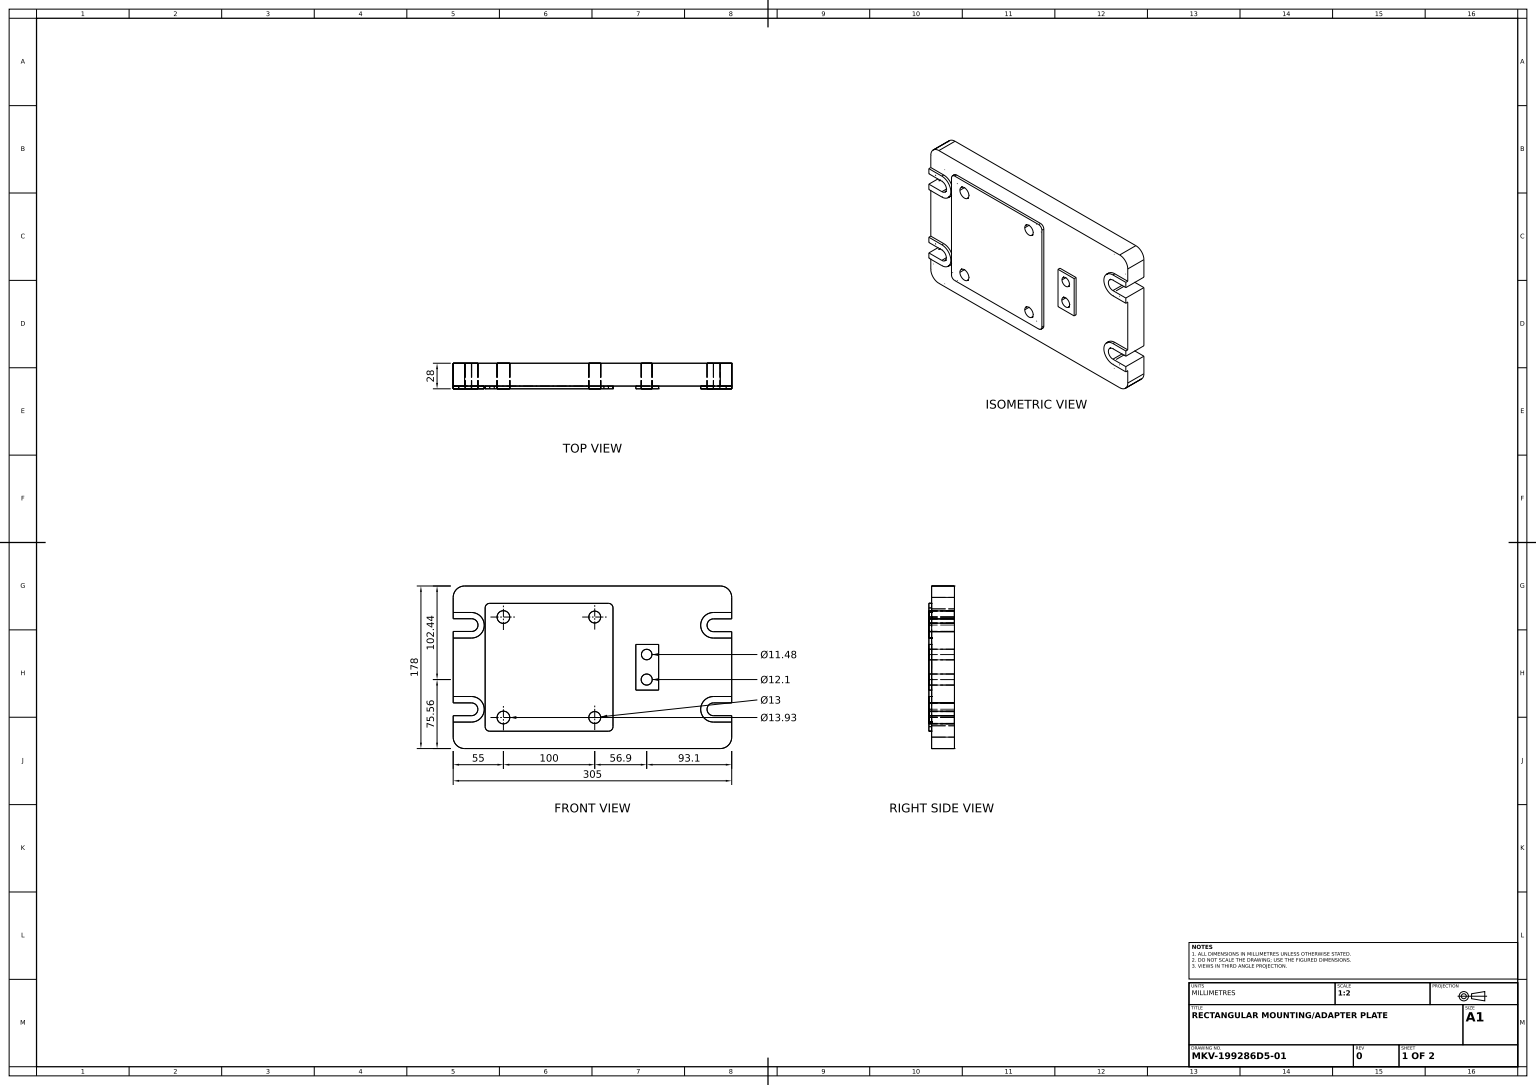
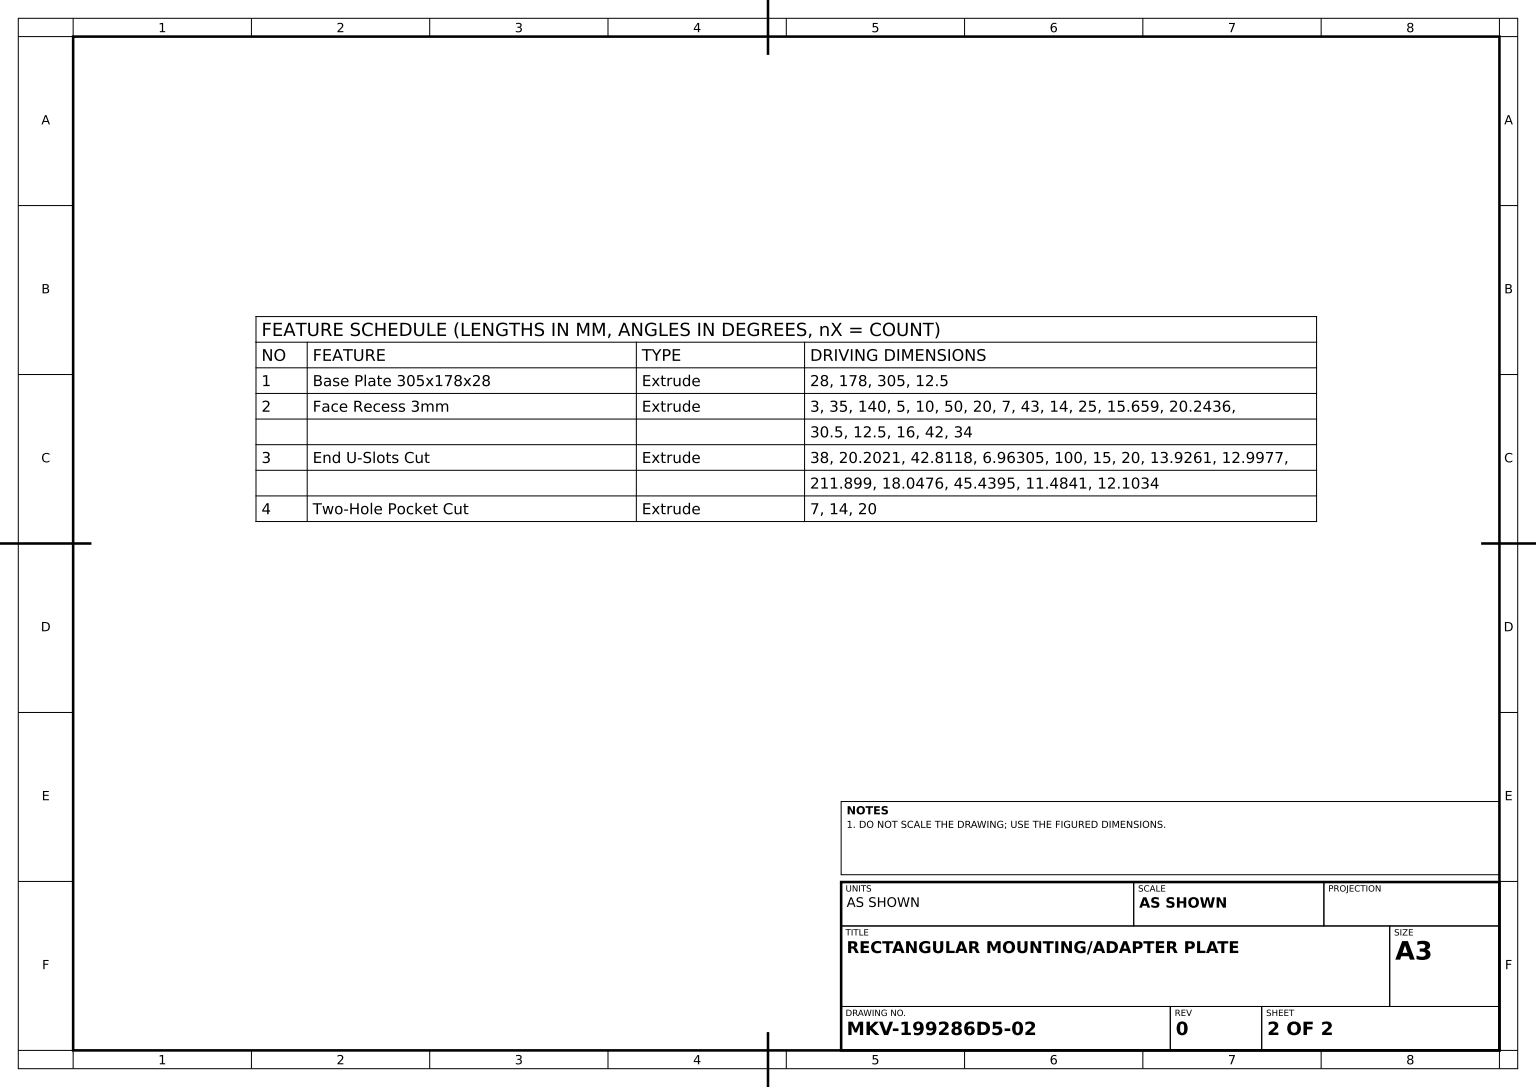
solid
v1 (152.5,53,14)
v2 (152.5,60,14)
e1 v1 v2 LINE
v3 (152.5,53,-14)
e2 v3 v1 LINE
v4 (152.5,76.5,-14)
e3 v3 v4 LINE
v5 (152.5,76.5,11)
e4 v5 v4 LINE
v6 (152.5,60,11)
e5 v6 v5 LINE
e6 v6 v2 LINE
face PLANE(AX(P(152.5,76.5,14),D(-1,0,0),D(0,0,1))) rev [-e1 -e2 e3 -e4 -e5 e6]
v7 (132.5,-53,-14)
v8 (152.5,-53,-14)
e7 v7 v8 LINE
v9 (132.5,-53,14)
e8 v7 v9 LINE
v10 (152.5,-53,14)
e9 v9 v10 LINE
e10 v8 v10 LINE
face PLANE(AX(P(152.5,-53,-14),D(0,-1,0),D(0,0,-1))) rev [-e7 e8 e9 -e10]
v11 (8.998844,-55,-14)
v12 (8.998844,-55,14)
e11 v11 v12 LINE
v13 (-3.998844,-55,14)
e12 v13 v12 CIRCLE(AX(P(2.5,-55,14),D(0,0,-1),D(1,0,0)),6.498844)
v14 (-3.998844,-55,-14)
e13 v14 v13 LINE
e14 v14 v11 CIRCLE(AX(P(2.5,-55,-14),D(0,0,-1),D(1,0,0)),6.498844)
face CYL(AX(P(2.5,-55,-24),D(0,0,1),D(1,0,0)),6.498844) rev [e11 -e12 -e13 e14]
v15 (152.5,32,14)
v16 (152.5,39,14)
e15 v15 v16 LINE
v17 (132.5,39,14)
e16 v17 v16 LINE
v18 (132.5,53,14)
e17 v18 v17 CIRCLE(AX(P(132.5,46,14),D(0,0,1),D(1,0,0)),7)
e18 v1 v18 LINE
v19 (132.5,60,14)
e19 v2 v19 LINE
v20 (132.5,32,14)
e20 v19 v20 CIRCLE(AX(P(132.5,46,14),D(0,0,1),D(1,0,0)),14)
e21 v15 v20 LINE
face PLANE(AX(P(-140,-76.5,14),D(0,0,1),D(1,0,0))) [e15 -e16 -e17 -e18 e1 e19 e20 -e21]
v21 (-125.33485,46.188213,-14)
v22 (-125.33485,46.188213,14)
e22 v21 v22 LINE
v23 (-132.297898,53.151261,14)
e23 v23 v22 CIRCLE(AX(P(-132.297898,46.188213,14),D(0,0,-1),D(1,0,0)),6.963047)
v24 (-132.297898,53.151261,-14)
e24 v24 v23 LINE
e25 v24 v21 CIRCLE(AX(P(-132.297898,46.188213,-14),D(0,0,-1),D(1,0,0)),6.963047)
face CYL(AX(P(-132.297898,46.188213,-24),D(0,0,1),D(1,0,0)),6.963047) rev [e22 -e23 -e24 e25]
v25 (-140,-89,11)
v26 (-140,-89,-14)
e26 v25 v26 LINE
v27 (-152.5,-76.5,11)
e27 v27 v25 CIRCLE(AX(P(-140,-76.5,11),D(0,0,1),D(1,0,0)),12.5)
v28 (-152.5,-76.5,-14)
e28 v27 v28 LINE
e29 v28 v26 CIRCLE(AX(P(-140,-76.5,-14),D(0,0,1),D(1,0,0)),12.5)
face CYL(AX(P(-140,-76.5,14),D(0,0,-1),D(-1,0,0)),12.5) [-e26 -e27 e28 e29]
v29 (-152.5,32,11)
v30 (-152.5,32,14)
e30 v29 v30 LINE
v31 (-152.5,39.225166,14)
e31 v31 v30 LINE
v32 (-152.5,39.225166,-14)
e32 v32 v31 LINE
v33 (-152.5,-39,-14)
e33 v32 v33 LINE
v34 (-152.5,-39,14)
e34 v33 v34 LINE
v35 (-152.5,-32,14)
e35 v35 v34 LINE
v36 (-152.5,-32,11)
e36 v36 v35 LINE
e37 v29 v36 LINE
face PLANE(AX(P(-152.5,76.5,14),D(1,0,0),D(0,0,-1))) rev [e30 -e31 -e32 e33 e34 -e35 -e36 -e37]
v37 (-104.463047,55,-14)
v38 (-104.463047,55,14)
e38 v37 v38 LINE
v39 (-90.536953,55,14)
e39 v38 v39 CIRCLE(AX(P(-97.5,55,14),D(0,0,1),D(1,0,0)),6.963047)
v40 (-90.536953,55,-14)
e40 v40 v39 LINE
e41 v37 v40 CIRCLE(AX(P(-97.5,55,-14),D(0,0,1),D(1,0,0)),6.963047)
face CYL(AX(P(-97.5,55,-24),D(0,0,1),D(1,0,0)),6.963047) rev [e38 e39 -e40 -e41]
v41 (-152.5,60,11)
v42 (-152.5,60,14)
e42 v41 v42 LINE
v43 (-152.5,76.5,11)
e43 v43 v41 LINE
v44 (-152.5,76.5,-14)
e44 v43 v44 LINE
v45 (-152.5,53.151261,-14)
e45 v44 v45 LINE
v46 (-152.5,53.151261,14)
e46 v45 v46 LINE
e47 v42 v46 LINE
face PLANE(AX(P(-152.5,76.5,14),D(1,0,0),D(0,0,-1))) rev [-e42 -e43 e44 e45 e46 -e47]
v47 (-132.5,32,11)
e48 v29 v47 LINE
v48 (-132.5,32,14)
e49 v47 v48 LINE
e50 v30 v48 LINE
face PLANE(AX(P(0,32,11),D(0,-1,0),D(0,0,-1))) [e48 e49 -e50 -e30]
v49 (132.5,-32,11)
v50 (132.5,-60,11)
e51 v49 v50 CIRCLE(AX(P(132.5,-46,11),D(0,0,1),D(1,0,0)),14)
v51 (132.5,-60,14)
e52 v50 v51 LINE
v52 (132.5,-32,14)
e53 v52 v51 CIRCLE(AX(P(132.5,-46,14),D(0,0,1),D(1,0,0)),14)
e54 v49 v52 LINE
face CYL(AX(P(132.5,-46,11),D(0,0,1),D(1,0,0)),14) [e51 e52 -e53 -e54]
v53 (-112.5,-70,11)
v54 (-112.5,-70,14)
e55 v53 v54 LINE
v55 (17.5,-70,11)
e56 v53 v55 LINE
v56 (17.5,-70,14)
e57 v55 v56 LINE
e58 v54 v56 LINE
face PLANE(AX(P(0,-70,11),D(0,-1,0),D(0,0,-1))) [-e55 e56 e57 -e58]
v57 (65.450566,-13.439495,-14)
v58 (53.347171,-13.439495,-14)
e59 v57 v58 CIRCLE(AX(P(59.398869,-13.439495,-14),D(0,0,1),D(1,0,0)),6.051697)
v59 (65.450566,-13.439495,14)
e60 v57 v59 LINE
v60 (53.347171,-13.439495,14)
e61 v59 v60 CIRCLE(AX(P(59.398869,-13.439495,14),D(0,0,1),D(1,0,0)),6.051697)
e62 v58 v60 LINE
face CYL(AX(P(59.398869,-13.439495,-24),D(0,0,1),D(1,0,0)),6.051697) rev [-e59 e60 e61 -e62]
v61 (-152.5,-60,14)
v62 (-132.5,-60,14)
e63 v61 v62 LINE
v63 (-152.5,-60,11)
e64 v63 v61 LINE
v64 (-132.5,-60,11)
e65 v63 v64 LINE
e66 v64 v62 LINE
face PLANE(AX(P(0,-60,11),D(0,-1,0),D(0,0,-1))) [-e63 -e64 e65 e66]
v65 (47.5,-25,11)
v66 (47.5,-25,14)
e67 v65 v66 LINE
v67 (47.5,25,14)
e68 v67 v66 LINE
v68 (47.5,25,11)
e69 v68 v67 LINE
e70 v68 v65 LINE
face PLANE(AX(P(47.5,0,11),D(-1,0,0),D(0,-1,0))) [e67 -e68 -e69 e70]
e71 v58 v57 CIRCLE(AX(P(59.398869,-13.439495,-14),D(0,0,1),D(1,0,0)),6.051697)
e72 v60 v59 CIRCLE(AX(P(59.398869,-13.439495,14),D(0,0,1),D(1,0,0)),6.051697)
face CYL(AX(P(59.398869,-13.439495,-24),D(0,0,1),D(1,0,0)),6.051697) rev [-e60 -e71 e62 e72]
v69 (-152.5,-53,14)
v70 (-132.5,-53,14)
e73 v69 v70 LINE
e74 v69 v61 LINE
v71 (-118.5,-46,14)
e75 v71 v62 CIRCLE(AX(P(-132.5,-46,14),D(0,0,-1),D(1,0,0)),14)
v72 (-132.5,-32,14)
e76 v72 v71 CIRCLE(AX(P(-132.5,-46,14),D(0,0,-1),D(1,0,0)),14)
e77 v35 v72 LINE
v73 (-132.5,-39,14)
e78 v73 v34 LINE
v74 (-125.5,-46,14)
e79 v74 v73 CIRCLE(AX(P(-132.5,-46,14),D(0,0,1),D(1,0,0)),7)
e80 v70 v74 CIRCLE(AX(P(-132.5,-46,14),D(0,0,1),D(1,0,0)),7)
face PLANE(AX(P(-140,-76.5,14),D(0,0,1),D(1,0,0))) [-e73 e74 e63 -e75 -e76 -e77 e35 -e78 -e79 -e80]
v75 (-90.536953,-55,14)
v76 (-104.463047,-55,14)
e81 v75 v76 CIRCLE(AX(P(-97.5,-55,14),D(0,0,-1),D(-1,0,0)),6.963047)
v77 (-90.536953,-55,-14)
e82 v77 v75 LINE
v78 (-104.463047,-55,-14)
e83 v77 v78 CIRCLE(AX(P(-97.5,-55,-14),D(0,0,-1),D(1,0,0)),6.963047)
e84 v78 v76 LINE
face CYL(AX(P(-97.5,-55,-24),D(0,0,1),D(1,0,0)),6.963047) rev [-e81 -e82 e83 e84]
v79 (8.998844,55,-14)
v80 (-3.998844,55,-14)
e85 v79 v80 CIRCLE(AX(P(2.5,55,-14),D(0,0,1),D(1,0,0)),6.498844)
e86 v80 v79 CIRCLE(AX(P(2.5,55,-14),D(0,0,1),D(1,0,0)),6.498844)
e87 v40 v37 CIRCLE(AX(P(-97.5,55,-14),D(0,0,1),D(1,0,0)),6.963047)
e88 v11 v14 CIRCLE(AX(P(2.5,-55,-14),D(0,0,-1),D(1,0,0)),6.498844)
v81 (-132.297898,39.225166,-14)
e89 v81 v32 LINE
e90 v21 v81 CIRCLE(AX(P(-132.297898,46.188213,-14),D(0,0,-1),D(1,0,0)),6.963047)
e91 v45 v24 LINE
v82 (-140,89,-14)
e92 v82 v44 CIRCLE(AX(P(-140,76.5,-14),D(0,0,1),D(1,0,0)),12.5)
v83 (140,89,-14)
e93 v83 v82 LINE
e94 v4 v83 CIRCLE(AX(P(140,76.5,-14),D(0,0,1),D(-1,0,0)),12.5)
v84 (132.5,53,-14)
e95 v3 v84 LINE
v85 (132.5,39,-14)
e96 v84 v85 CIRCLE(AX(P(132.5,46,-14),D(0,0,1),D(-1,0,0)),7)
v86 (152.5,39,-14)
e97 v85 v86 LINE
v87 (152.5,-39,-14)
e98 v87 v86 LINE
v88 (132.5,-39,-14)
e99 v87 v88 LINE
e100 v88 v7 CIRCLE(AX(P(132.5,-46,-14),D(0,0,1),D(1,0,0)),7)
v89 (152.5,-76.5,-14)
e101 v89 v8 LINE
v90 (140,-89,-14)
e102 v90 v89 CIRCLE(AX(P(140,-76.5,-14),D(0,0,1),D(1,0,0)),12.5)
e103 v26 v90 LINE
v91 (-152.5,-53,-14)
e104 v91 v28 LINE
v92 (-132.5,-53,-14)
e105 v91 v92 LINE
v93 (-125.5,-46,-14)
e106 v92 v93 CIRCLE(AX(P(-132.5,-46,-14),D(0,0,1),D(-1,0,0)),7)
v94 (-132.5,-39,-14)
e107 v93 v94 CIRCLE(AX(P(-132.5,-46,-14),D(0,0,1),D(-1,0,0)),7)
e108 v94 v33 LINE
e109 v78 v77 CIRCLE(AX(P(-97.5,-55,-14),D(0,0,-1),D(1,0,0)),6.963047)
v95 (65.140896,13.952399,-14)
v96 (53.656841,13.952399,-14)
e110 v95 v96 CIRCLE(AX(P(59.398869,13.952399,-14),D(0,0,1),D(1,0,0)),5.742028)
e111 v96 v95 CIRCLE(AX(P(59.398869,13.952399,-14),D(0,0,1),D(1,0,0)),5.742028)
face PLANE(AX(P(-140,-76.5,-14),D(0,0,1),D(1,0,0))) rev [e85 e86] [e41 e87] [-e88 -e14] [-e33 -e89 -e90 -e25 -e91 -e45 -e92 -e93 -e94 -e3 e95 e96 e97 -e98 e99 e100 e7 -e101 -e102 -e103 -e29 -e104 e105 e106 e107 e108] [-e83 -e109] [e110 e111] [e71 e59]
e112 v12 v13 CIRCLE(AX(P(2.5,-55,14),D(0,0,-1),D(1,0,0)),6.498844)
face CYL(AX(P(2.5,-55,-24),D(0,0,1),D(1,0,0)),6.498844) rev [e13 -e112 -e11 e88]
v97 (-117.5,-65,14)
e113 v97 v54 CIRCLE(AX(P(-112.5,-65,14),D(0,0,1),D(1,0,0)),5)
v98 (-117.5,-65,11)
e114 v98 v97 LINE
e115 v98 v53 CIRCLE(AX(P(-112.5,-65,11),D(0,0,1),D(1,0,0)),5)
face CYL(AX(P(-112.5,-65,11),D(0,0,1),D(1,0,0)),5) [-e113 -e114 e115 e55]
v99 (-132.297898,39.225166,14)
e116 v99 v31 LINE
e117 v81 v99 LINE
face PLANE(AX(P(0,39.225166,-24),D(0,1,0),D(0,0,1))) [e89 e32 -e116 -e117]
v100 (-132.5,-32,11)
v101 (-118.5,-46,11)
e118 v100 v101 CIRCLE(AX(P(-132.5,-46,11),D(0,0,-1),D(1,0,0)),14)
e119 v100 v72 LINE
e120 v101 v71 LINE
face CYL(AX(P(-132.5,-46,11),D(0,0,1),D(1,0,0)),14) [-e118 e119 e76 -e120]
v102 (132.5,60,11)
e121 v6 v102 LINE
e122 v102 v19 LINE
face PLANE(AX(P(0,60,11),D(0,1,0),D(-1,0,0))) [e121 e122 -e19 -e6]
v103 (-118.5,46,11)
e123 v103 v47 CIRCLE(AX(P(-132.5,46,11),D(0,0,-1),D(1,0,0)),14)
v104 (-118.5,46,14)
e124 v103 v104 LINE
e125 v104 v48 CIRCLE(AX(P(-132.5,46,14),D(0,0,-1),D(1,0,0)),14)
face CYL(AX(P(-132.5,46,11),D(0,0,1),D(1,0,0)),14) [-e49 -e123 e124 e125]
v105 (132.5,-39,14)
e126 v88 v105 LINE
e127 v105 v9 CIRCLE(AX(P(132.5,-46,14),D(0,0,1),D(1,0,0)),7)
face CYL(AX(P(132.5,-46,-14),D(0,0,1),D(1,0,0)),7) rev [-e100 e126 e127 -e8]
v106 (152.5,-32,14)
e128 v106 v52 LINE
v107 (152.5,-32,11)
e129 v107 v106 LINE
e130 v107 v49 LINE
face PLANE(AX(P(0,-32,11),D(0,1,0),D(0,0,1))) [-e128 -e129 e130 e54]
v108 (152.5,-39,14)
e131 v108 v105 LINE
e132 v108 v106 LINE
v109 (152.5,-60,14)
e133 v109 v51 LINE
e134 v109 v10 LINE
face PLANE(AX(P(-140,-76.5,14),D(0,0,1),D(1,0,0))) [-e127 -e131 e132 e128 e53 -e133 e134 -e9]
v110 (22.5,-65,14)
e135 v56 v110 CIRCLE(AX(P(17.5,-65,14),D(0,0,1),D(1,0,0)),5)
v111 (22.5,-65,11)
e136 v55 v111 CIRCLE(AX(P(17.5,-65,11),D(0,0,1),D(1,0,0)),5)
e137 v111 v110 LINE
face CYL(AX(P(17.5,-65,11),D(0,0,1),D(1,0,0)),5) [-e135 -e57 e136 e137]
v112 (-132.5,60,11)
v113 (-132.5,60,14)
e138 v112 v113 LINE
e139 v41 v112 LINE
e140 v42 v113 LINE
face PLANE(AX(P(0,60,11),D(0,-1,0),D(0,0,-1))) rev [-e138 -e139 e42 e140]
v114 (53.656841,13.952399,14)
v115 (65.140896,13.952399,14)
e141 v114 v115 CIRCLE(AX(P(59.398869,13.952399,14),D(0,0,1),D(1,0,0)),5.742028)
e142 v95 v115 LINE
e143 v96 v114 LINE
face CYL(AX(P(59.398869,13.952399,-24),D(0,0,1),D(1,0,0)),5.742028) rev [e141 -e142 -e111 e143]
v116 (72.5,-25,11)
v117 (72.5,-25,14)
e144 v116 v117 LINE
v118 (72.5,25,11)
e145 v118 v116 LINE
v119 (72.5,25,14)
e146 v118 v119 LINE
e147 v119 v117 LINE
face PLANE(AX(P(72.5,0,11),D(-1,0,0),D(0,0,1))) rev [-e144 -e145 e146 e147]
e148 v22 v99 CIRCLE(AX(P(-132.297898,46.188213,14),D(0,0,-1),D(1,0,0)),6.963047)
face CYL(AX(P(-132.297898,46.188213,-24),D(0,0,1),D(1,0,0)),6.963047) rev [e117 -e148 -e22 e90]
e149 v85 v17 LINE
e150 v84 v18 LINE
face CYL(AX(P(132.5,46,-14),D(0,0,1),D(1,0,0)),7) rev [-e149 -e96 e150 e17]
v120 (8.998844,55,14)
e151 v79 v120 LINE
v121 (-3.998844,55,14)
e152 v120 v121 CIRCLE(AX(P(2.5,55,14),D(0,0,1),D(1,0,0)),6.498844)
e153 v80 v121 LINE
face CYL(AX(P(2.5,55,-24),D(0,0,1),D(1,0,0)),6.498844) rev [e151 e152 -e153 -e85]
e154 v115 v114 CIRCLE(AX(P(59.398869,13.952399,14),D(0,0,1),D(1,0,0)),5.742028)
e155 v67 v119 LINE
e156 v66 v117 LINE
face PLANE(AX(P(-140,-76.5,14),D(0,0,1),D(1,0,0))) [-e61 -e72] [-e141 -e154] [-e147 -e155 e68 e156]
e157 v39 v38 CIRCLE(AX(P(-97.5,55,14),D(0,0,1),D(1,0,0)),6.963047)
face CYL(AX(P(-97.5,55,-24),D(0,0,1),D(1,0,0)),6.963047) rev [e40 e157 -e38 -e87]
e158 v87 v108 LINE
face PLANE(AX(P(152.5,-39,-14),D(0,1,0),D(0,0,1))) rev [e131 -e126 -e99 e158]
face PLANE(AX(P(152.5,53,-14),D(0,1,0),D(0,0,1))) rev [-e150 -e95 e2 e18]
e159 v101 v64 CIRCLE(AX(P(-132.5,-46,11),D(0,0,-1),D(1,0,0)),14)
face CYL(AX(P(-132.5,-46,11),D(0,0,1),D(1,0,0)),14) [e120 e75 -e66 -e159]
e160 v63 v27 LINE
e161 v91 v69 LINE
face PLANE(AX(P(-152.5,76.5,14),D(1,0,0),D(0,0,-1))) rev [-e160 e64 -e74 -e161 e104 -e28]
e162 v65 v116 LINE
face PLANE(AX(P(0,-25,11),D(0,-1,0),D(1,0,0))) [-e156 -e67 e162 e144]
e163 v112 v103 CIRCLE(AX(P(-132.5,46,11),D(0,0,-1),D(1,0,0)),14)
e164 v113 v104 CIRCLE(AX(P(-132.5,46,14),D(0,0,-1),D(1,0,0)),14)
face CYL(AX(P(-132.5,46,11),D(0,0,1),D(1,0,0)),14) [-e124 -e163 e138 e164]
v122 (-140,89,11)
e165 v122 v82 LINE
v123 (140,89,11)
e166 v123 v122 LINE
e167 v123 v83 LINE
face PLANE(AX(P(-140,89,14),D(0,-1,0),D(0,0,-1))) rev [e93 -e165 -e166 e167]
e168 v46 v23 LINE
face PLANE(AX(P(-140,-76.5,14),D(0,0,1),D(1,0,0))) [e23 e148 e116 e31 e50 -e125 -e164 -e140 e47 e168]
v124 (140,-89,11)
e169 v124 v90 LINE
e170 v25 v124 LINE
face PLANE(AX(P(-140,-89,14),D(0,1,0),D(0,0,1))) rev [-e169 -e170 e26 e103]
v125 (132.5,32,11)
e171 v102 v125 CIRCLE(AX(P(132.5,46,11),D(0,0,1),D(1,0,0)),14)
e172 v125 v20 LINE
face CYL(AX(P(132.5,46,11),D(0,0,1),D(1,0,0)),14) [e171 e172 -e20 -e122]
e173 v92 v70 LINE
face PLANE(AX(P(-152.5,-53,-14),D(0,-1,0),D(0,0,-1))) rev [-e173 -e105 e161 e73]
v126 (-117.5,65,11)
e174 v126 v98 LINE
v127 (-117.5,65,14)
e175 v127 v97 LINE
e176 v126 v127 LINE
face PLANE(AX(P(-117.5,0,11),D(-1,0,0),D(0,-1,0))) [e174 e114 -e175 -e176]
e177 v122 v43 CIRCLE(AX(P(-140,76.5,11),D(0,0,1),D(1,0,0)),12.5)
face CYL(AX(P(-140,76.5,14),D(0,0,-1),D(-1,0,0)),12.5) [e92 -e44 -e177 e165]
face CYL(AX(P(59.398869,13.952399,-24),D(0,0,1),D(1,0,0)),5.742028) rev [e154 -e143 -e110 e142]
v128 (17.5,70,11)
v129 (17.5,70,14)
e178 v128 v129 LINE
v130 (-112.5,70,11)
e179 v130 v128 LINE
v131 (-112.5,70,14)
e180 v130 v131 LINE
e181 v131 v129 LINE
face PLANE(AX(P(0,70,11),D(0,-1,0),D(0,0,-1))) rev [-e178 -e179 e180 e181]
v132 (22.5,65,11)
e182 v128 v132 CIRCLE(AX(P(17.5,65,11),D(0,0,-1),D(1,0,0)),5)
v133 (22.5,65,14)
e183 v129 v133 CIRCLE(AX(P(17.5,65,14),D(0,0,-1),D(1,0,0)),5)
e184 v132 v133 LINE
face CYL(AX(P(17.5,65,11),D(0,0,1),D(1,0,0)),5) [-e182 e178 e183 -e184]
v134 (152.5,32,11)
e185 v134 v125 LINE
e186 v134 v15 LINE
face PLANE(AX(P(0,32,11),D(0,1,0),D(0,0,1))) rev [e21 -e172 -e185 e186]
e187 v130 v126 CIRCLE(AX(P(-112.5,65,11),D(0,0,1),D(1,0,0)),5)
e188 v131 v127 CIRCLE(AX(P(-112.5,65,14),D(0,0,1),D(1,0,0)),5)
face CYL(AX(P(-112.5,65,11),D(0,0,1),D(1,0,0)),5) [e187 e176 -e188 -e180]
e189 v76 v75 CIRCLE(AX(P(-97.5,-55,14),D(0,0,-1),D(-1,0,0)),6.963047)
e190 v133 v110 LINE
e191 v121 v120 CIRCLE(AX(P(2.5,55,14),D(0,0,1),D(1,0,0)),6.498844)
face PLANE(AX(P(-140,-76.5,14),D(0,0,1),D(1,0,0))) [e81 e189] [e135 -e190 -e183 -e181 e188 e175 e113 e58] [-e152 -e191] [-e39 -e157] [e12 e112]
e192 v132 v111 LINE
face PLANE(AX(P(22.5,0,11),D(-1,0,0),D(0,-1,0))) rev [-e192 e184 e190 -e137]
e193 v68 v118 LINE
face PLANE(AX(P(0,25,11),D(0,-1,0),D(1,0,0))) rev [-e193 e69 e155 -e146]
e194 v93 v74 LINE
face CYL(AX(P(-132.5,-46,-14),D(0,0,1),D(1,0,0)),7) rev [-e194 -e106 e173 e80]
face CYL(AX(P(2.5,55,-24),D(0,0,1),D(1,0,0)),6.498844) rev [-e86 e153 e191 -e151]
face CYL(AX(P(-97.5,-55,-24),D(0,0,1),D(1,0,0)),6.963047) rev [e82 -e189 -e84 e109]
e195 v86 v16 LINE
e196 v107 v134 LINE
face PLANE(AX(P(152.5,76.5,14),D(-1,0,0),D(0,0,1))) rev [e129 -e132 -e158 e98 e195 -e15 -e186 -e196]
v135 (152.5,-60,11)
e197 v135 v109 LINE
v136 (152.5,-76.5,11)
e198 v136 v135 LINE
e199 v136 v89 LINE
face PLANE(AX(P(152.5,76.5,14),D(-1,0,0),D(0,0,1))) rev [e101 e10 -e134 -e197 -e198 e199]
e200 v94 v73 LINE
face CYL(AX(P(-132.5,-46,-14),D(0,0,1),D(1,0,0)),7) rev [-e107 e194 e79 -e200]
e201 v36 v100 LINE
face PLANE(AX(P(0,-32,11),D(0,-1,0),D(0,0,-1))) rev [-e119 -e201 e36 e77]
face PLANE(AX(P(152.5,39,-14),D(0,-1,0),D(0,0,-1))) rev [-e97 e149 e16 -e195]
e202 v5 v123 CIRCLE(AX(P(140,76.5,11),D(0,0,1),D(1,0,0)),12.5)
face CYL(AX(P(140,76.5,14),D(0,0,-1),D(-1,0,0)),12.5) [-e202 e4 e94 -e167]
face PLANE(AX(P(0,53.151261,-24),D(0,-1,0),D(0,0,-1))) [e24 -e168 -e46 e91]
e203 v124 v136 CIRCLE(AX(P(140,-76.5,11),D(0,0,1),D(1,0,0)),12.5)
e204 v135 v50 LINE
face PLANE(AX(P(0,0,11),D(0,0,1),D(1,0,0))) [-e56 -e115 -e174 -e187 e179 e182 e192 -e136] [e5 e202 e166 e177 e43 e139 e163 e123 -e48 e37 e201 e118 e159 -e65 e160 e27 e170 e203 e198 e204 -e51 -e130 e196 e185 -e171 -e121] [e193 e145 -e162 -e70]
face PLANE(AX(P(-152.5,-39,-14),D(0,1,0),D(0,0,1))) rev [e78 -e34 -e108 e200]
face PLANE(AX(P(0,-60,11),D(0,1,0),D(0,0,1))) rev [e133 -e52 -e204 e197]
face CYL(AX(P(140,-76.5,14),D(0,0,-1),D(-1,0,0)),12.5) [-e199 -e203 e169 e102]
